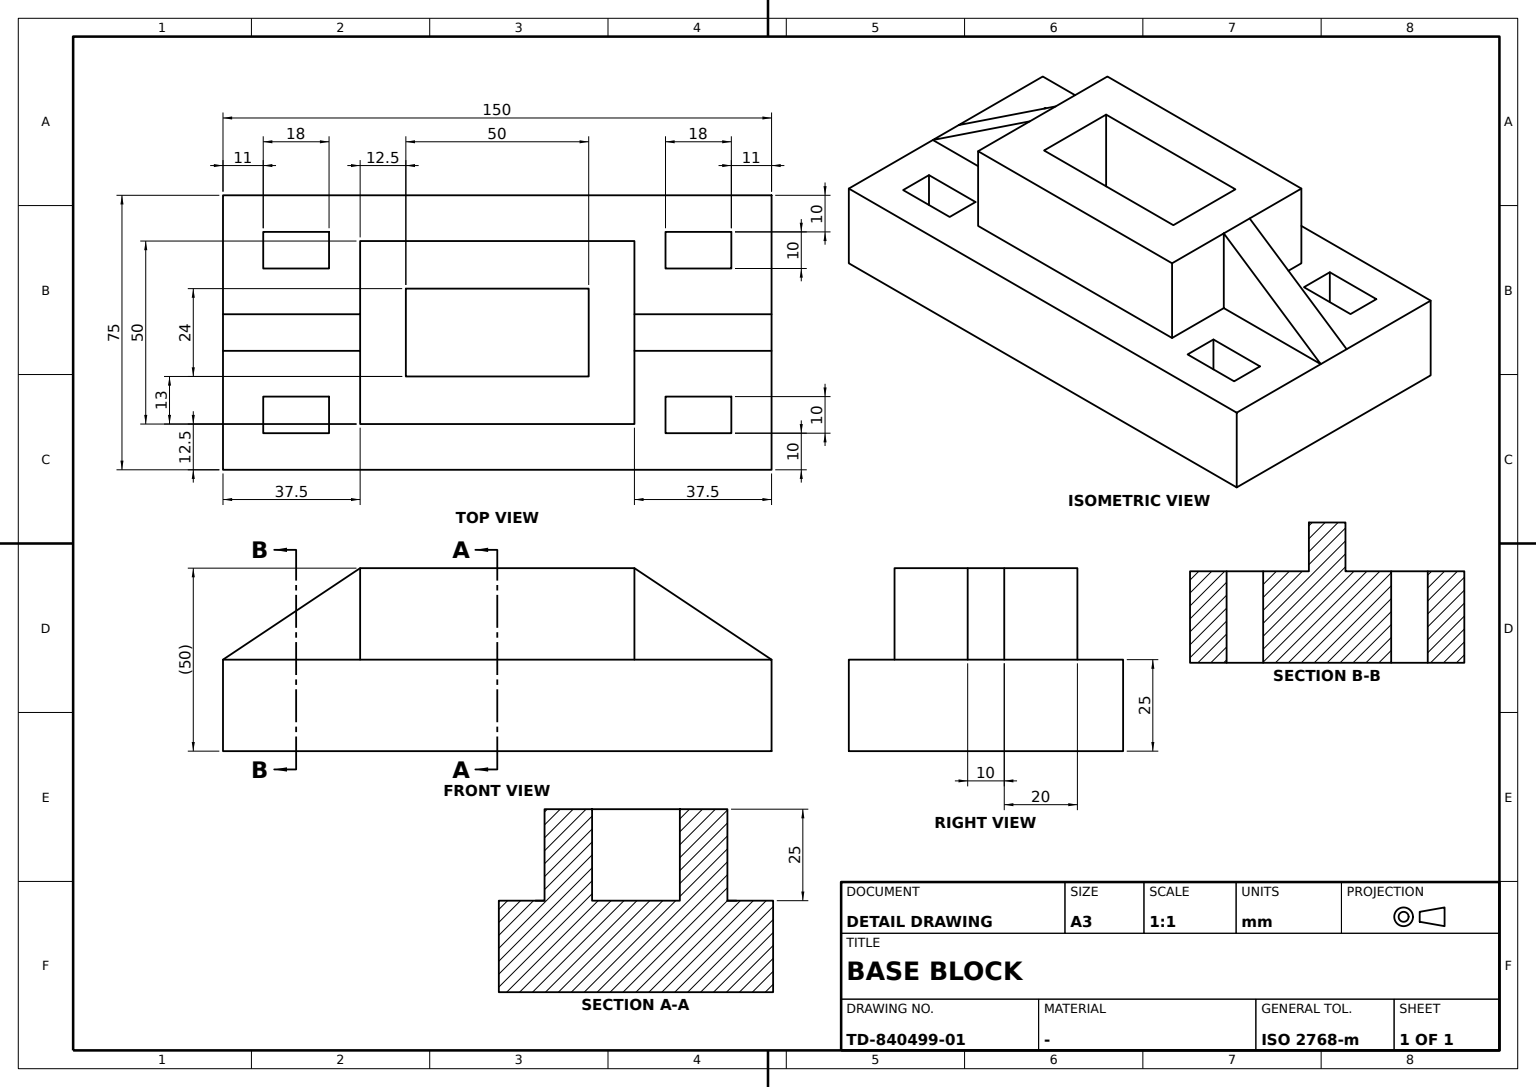
ISO-10303-21;
HEADER;
FILE_DESCRIPTION((''),'2;1');
FILE_NAME('','',(''),(''),'','','');
FILE_SCHEMA(('AUTOMOTIVE_DESIGN'));
ENDSEC;
DATA;
#1=APPLICATION_CONTEXT('');
#2=PRODUCT_CONTEXT('',#1,'mechanical');
#3=PRODUCT('','','',(#2));
#4=PRODUCT_DEFINITION_FORMATION('','',#3);
#5=PRODUCT_DEFINITION_CONTEXT('',#1,'design');
#6=PRODUCT_DEFINITION('','',#4,#5);
#7=PRODUCT_DEFINITION_SHAPE('','',#6);
#8=(LENGTH_UNIT()NAMED_UNIT(*)SI_UNIT(.MILLI.,.METRE.));
#9=(NAMED_UNIT(*)PLANE_ANGLE_UNIT()SI_UNIT($,.RADIAN.));
#10=(NAMED_UNIT(*)SI_UNIT($,.STERADIAN.)SOLID_ANGLE_UNIT());
#11=UNCERTAINTY_MEASURE_WITH_UNIT(LENGTH_MEASURE(0.005),#8,'distance_accuracy_value','');
#12=(GEOMETRIC_REPRESENTATION_CONTEXT(3)GLOBAL_UNCERTAINTY_ASSIGNED_CONTEXT((#11))GLOBAL_UNIT_ASSIGNED_CONTEXT((#8,#9,#10))REPRESENTATION_CONTEXT('',''));
#13=CARTESIAN_POINT('',(-46.,17.5,25.));
#14=VERTEX_POINT('',#13);
#15=CARTESIAN_POINT('',(-64.,17.5,25.));
#16=VERTEX_POINT('',#15);
#17=CARTESIAN_POINT('',(64.,17.5,25.));
#18=DIRECTION('',(-1.,0.,0.));
#19=VECTOR('',#18,1000.);
#20=LINE('',#17,#19);
#21=EDGE_CURVE('',#14,#16,#20,.T.);
#22=ORIENTED_EDGE('',*,*,#21,.F.);
#23=CARTESIAN_POINT('',(-46.,17.5,0.));
#24=VERTEX_POINT('',#23);
#25=DIRECTION('',(0.,0.,-1.));
#26=VECTOR('',#25,1000.);
#27=LINE('',#13,#26);
#28=EDGE_CURVE('',#14,#24,#27,.T.);
#29=ORIENTED_EDGE('',*,*,#28,.T.);
#30=CARTESIAN_POINT('',(-64.,17.5,0.));
#31=VERTEX_POINT('',#30);
#32=CARTESIAN_POINT('',(64.,17.5,0.));
#33=LINE('',#32,#19);
#34=EDGE_CURVE('',#24,#31,#33,.T.);
#35=ORIENTED_EDGE('',*,*,#34,.T.);
#36=LINE('',#15,#26);
#37=EDGE_CURVE('',#16,#31,#36,.T.);
#38=ORIENTED_EDGE('',*,*,#37,.F.);
#39=EDGE_LOOP('',(#22,#29,#35,#38));
#40=FACE_BOUND('',#39,.T.);
#41=DIRECTION('',(0.,-1.,0.));
#42=AXIS2_PLACEMENT_3D('',#17,#41,#18);
#43=PLANE('',#42);
#44=ADVANCED_FACE('',(#40),#43,.F.);
#45=VERTEX_POINT('',#17);
#46=CARTESIAN_POINT('',(46.,17.5,25.));
#47=VERTEX_POINT('',#46);
#48=EDGE_CURVE('',#45,#47,#20,.T.);
#49=ORIENTED_EDGE('',*,*,#48,.F.);
#50=VERTEX_POINT('',#32);
#51=LINE('',#17,#26);
#52=EDGE_CURVE('',#45,#50,#51,.T.);
#53=ORIENTED_EDGE('',*,*,#52,.T.);
#54=CARTESIAN_POINT('',(46.,17.5,0.));
#55=VERTEX_POINT('',#54);
#56=EDGE_CURVE('',#50,#55,#33,.T.);
#57=ORIENTED_EDGE('',*,*,#56,.T.);
#58=LINE('',#46,#26);
#59=EDGE_CURVE('',#47,#55,#58,.T.);
#60=ORIENTED_EDGE('',*,*,#59,.F.);
#61=EDGE_LOOP('',(#49,#53,#57,#60));
#62=FACE_BOUND('',#61,.T.);
#63=ADVANCED_FACE('',(#62),#43,.F.);
#64=CARTESIAN_POINT('',(75.,37.5,0.));
#65=VERTEX_POINT('',#64);
#66=CARTESIAN_POINT('',(75.,37.5,25.));
#67=VERTEX_POINT('',#66);
#68=DIRECTION('',(0.,0.,1.));
#69=VECTOR('',#68,1000.);
#70=LINE('',#64,#69);
#71=EDGE_CURVE('',#65,#67,#70,.T.);
#72=ORIENTED_EDGE('',*,*,#71,.F.);
#73=CARTESIAN_POINT('',(-75.,37.5,0.));
#74=VERTEX_POINT('',#73);
#75=CARTESIAN_POINT('',(0.,37.5,0.));
#76=DIRECTION('',(1.,0.,0.));
#77=VECTOR('',#76,1000.);
#78=LINE('',#75,#77);
#79=EDGE_CURVE('',#74,#65,#78,.T.);
#80=ORIENTED_EDGE('',*,*,#79,.F.);
#81=CARTESIAN_POINT('',(-75.,37.5,25.));
#82=VERTEX_POINT('',#81);
#83=LINE('',#73,#69);
#84=EDGE_CURVE('',#74,#82,#83,.T.);
#85=ORIENTED_EDGE('',*,*,#84,.T.);
#86=CARTESIAN_POINT('',(0.,37.5,25.));
#87=LINE('',#86,#77);
#88=EDGE_CURVE('',#82,#67,#87,.T.);
#89=ORIENTED_EDGE('',*,*,#88,.T.);
#90=EDGE_LOOP('',(#72,#80,#85,#89));
#91=FACE_BOUND('',#90,.T.);
#92=AXIS2_PLACEMENT_3D('',#73,#41,#76);
#93=PLANE('',#92);
#94=ADVANCED_FACE('',(#91),#93,.F.);
#95=CARTESIAN_POINT('',(75.,-5.,25.));
#96=VERTEX_POINT('',#95);
#97=CARTESIAN_POINT('',(75.,5.,25.));
#98=VERTEX_POINT('',#97);
#99=DIRECTION('',(0.,1.,0.));
#100=VECTOR('',#99,1000.);
#101=LINE('',#66,#100);
#102=EDGE_CURVE('',#96,#98,#101,.T.);
#103=ORIENTED_EDGE('',*,*,#102,.T.);
#104=CARTESIAN_POINT('',(37.5,5.,50.));
#105=VERTEX_POINT('',#104);
#106=CARTESIAN_POINT('',(34.615385,5.,51.923077));
#107=DIRECTION('',(0.832050294,0.,-0.554700196));
#108=VECTOR('',#107,1000.);
#109=LINE('',#106,#108);
#110=EDGE_CURVE('',#105,#98,#109,.T.);
#111=ORIENTED_EDGE('',*,*,#110,.F.);
#112=CARTESIAN_POINT('',(37.5,-5.,50.));
#113=VERTEX_POINT('',#112);
#114=CARTESIAN_POINT('',(37.5,0.,50.));
#115=LINE('',#114,#100);
#116=EDGE_CURVE('',#113,#105,#115,.T.);
#117=ORIENTED_EDGE('',*,*,#116,.F.);
#118=CARTESIAN_POINT('',(34.615385,-5.,51.923077));
#119=LINE('',#118,#108);
#120=EDGE_CURVE('',#113,#96,#119,.T.);
#121=ORIENTED_EDGE('',*,*,#120,.T.);
#122=EDGE_LOOP('',(#103,#111,#117,#121));
#123=FACE_BOUND('',#122,.T.);
#124=DIRECTION('',(0.554700196,0.,0.832050294));
#125=AXIS2_PLACEMENT_3D('',#114,#124,#107);
#126=PLANE('',#125);
#127=ADVANCED_FACE('',(#123),#126,.T.);
#128=ORIENTED_EDGE('',*,*,#79,.T.);
#129=CARTESIAN_POINT('',(75.,-37.5,0.));
#130=VERTEX_POINT('',#129);
#131=CARTESIAN_POINT('',(75.,0.,0.));
#132=VECTOR('',#41,1000.);
#133=LINE('',#131,#132);
#134=EDGE_CURVE('',#65,#130,#133,.T.);
#135=ORIENTED_EDGE('',*,*,#134,.T.);
#136=CARTESIAN_POINT('',(-75.,-37.5,0.));
#137=VERTEX_POINT('',#136);
#138=CARTESIAN_POINT('',(0.,-37.5,0.));
#139=LINE('',#138,#19);
#140=EDGE_CURVE('',#130,#137,#139,.T.);
#141=ORIENTED_EDGE('',*,*,#140,.T.);
#142=CARTESIAN_POINT('',(-75.,0.,0.));
#143=LINE('',#142,#100);
#144=EDGE_CURVE('',#137,#74,#143,.T.);
#145=ORIENTED_EDGE('',*,*,#144,.T.);
#146=EDGE_LOOP('',(#128,#135,#141,#145));
#147=FACE_BOUND('',#146,.T.);
#148=CARTESIAN_POINT('',(64.,-27.5,0.));
#149=VERTEX_POINT('',#148);
#150=CARTESIAN_POINT('',(46.,-27.5,0.));
#151=VERTEX_POINT('',#150);
#152=LINE('',#148,#19);
#153=EDGE_CURVE('',#149,#151,#152,.T.);
#154=ORIENTED_EDGE('',*,*,#153,.F.);
#155=CARTESIAN_POINT('',(64.,-17.5,0.));
#156=VERTEX_POINT('',#155);
#157=CARTESIAN_POINT('',(64.,27.5,0.));
#158=LINE('',#157,#132);
#159=EDGE_CURVE('',#156,#149,#158,.T.);
#160=ORIENTED_EDGE('',*,*,#159,.F.);
#161=CARTESIAN_POINT('',(46.,-17.5,0.));
#162=VERTEX_POINT('',#161);
#163=LINE('',#161,#77);
#164=EDGE_CURVE('',#162,#156,#163,.T.);
#165=ORIENTED_EDGE('',*,*,#164,.F.);
#166=LINE('',#54,#100);
#167=EDGE_CURVE('',#151,#162,#166,.T.);
#168=ORIENTED_EDGE('',*,*,#167,.F.);
#169=EDGE_LOOP('',(#154,#160,#165,#168));
#170=FACE_BOUND('',#169,.T.);
#171=VERTEX_POINT('',#157);
#172=EDGE_CURVE('',#171,#50,#158,.T.);
#173=ORIENTED_EDGE('',*,*,#172,.F.);
#174=CARTESIAN_POINT('',(46.,27.5,0.));
#175=VERTEX_POINT('',#174);
#176=LINE('',#174,#77);
#177=EDGE_CURVE('',#175,#171,#176,.T.);
#178=ORIENTED_EDGE('',*,*,#177,.F.);
#179=EDGE_CURVE('',#55,#175,#166,.T.);
#180=ORIENTED_EDGE('',*,*,#179,.F.);
#181=ORIENTED_EDGE('',*,*,#56,.F.);
#182=EDGE_LOOP('',(#173,#178,#180,#181));
#183=FACE_BOUND('',#182,.T.);
#184=CARTESIAN_POINT('',(-46.,-17.5,0.));
#185=VERTEX_POINT('',#184);
#186=CARTESIAN_POINT('',(-46.,-27.5,0.));
#187=VERTEX_POINT('',#186);
#188=CARTESIAN_POINT('',(-46.,27.5,0.));
#189=LINE('',#188,#132);
#190=EDGE_CURVE('',#185,#187,#189,.T.);
#191=ORIENTED_EDGE('',*,*,#190,.F.);
#192=CARTESIAN_POINT('',(-64.,-17.5,0.));
#193=VERTEX_POINT('',#192);
#194=EDGE_CURVE('',#193,#185,#163,.T.);
#195=ORIENTED_EDGE('',*,*,#194,.F.);
#196=CARTESIAN_POINT('',(-64.,-27.5,0.));
#197=VERTEX_POINT('',#196);
#198=LINE('',#30,#100);
#199=EDGE_CURVE('',#197,#193,#198,.T.);
#200=ORIENTED_EDGE('',*,*,#199,.F.);
#201=EDGE_CURVE('',#187,#197,#152,.T.);
#202=ORIENTED_EDGE('',*,*,#201,.F.);
#203=EDGE_LOOP('',(#191,#195,#200,#202));
#204=FACE_BOUND('',#203,.T.);
#205=VERTEX_POINT('',#188);
#206=EDGE_CURVE('',#205,#24,#189,.T.);
#207=ORIENTED_EDGE('',*,*,#206,.F.);
#208=CARTESIAN_POINT('',(-64.,27.5,0.));
#209=VERTEX_POINT('',#208);
#210=EDGE_CURVE('',#209,#205,#176,.T.);
#211=ORIENTED_EDGE('',*,*,#210,.F.);
#212=EDGE_CURVE('',#31,#209,#198,.T.);
#213=ORIENTED_EDGE('',*,*,#212,.F.);
#214=ORIENTED_EDGE('',*,*,#34,.F.);
#215=EDGE_LOOP('',(#207,#211,#213,#214));
#216=FACE_BOUND('',#215,.T.);
#217=CARTESIAN_POINT('',(0.,0.,0.));
#218=AXIS2_PLACEMENT_3D('',#217,#68,#76);
#219=PLANE('',#218);
#220=ADVANCED_FACE('',(#147,#170,#183,#204,#216),#219,.F.);
#221=CARTESIAN_POINT('',(25.,-12.,50.));
#222=VERTEX_POINT('',#221);
#223=CARTESIAN_POINT('',(-25.,-12.,50.));
#224=VERTEX_POINT('',#223);
#225=CARTESIAN_POINT('',(0.,-12.,50.));
#226=LINE('',#225,#19);
#227=EDGE_CURVE('',#222,#224,#226,.T.);
#228=ORIENTED_EDGE('',*,*,#227,.T.);
#229=CARTESIAN_POINT('',(-25.,12.,50.));
#230=VERTEX_POINT('',#229);
#231=CARTESIAN_POINT('',(-25.,0.,50.));
#232=LINE('',#231,#100);
#233=EDGE_CURVE('',#224,#230,#232,.T.);
#234=ORIENTED_EDGE('',*,*,#233,.T.);
#235=CARTESIAN_POINT('',(25.,12.,50.));
#236=VERTEX_POINT('',#235);
#237=CARTESIAN_POINT('',(0.,12.,50.));
#238=LINE('',#237,#77);
#239=EDGE_CURVE('',#230,#236,#238,.T.);
#240=ORIENTED_EDGE('',*,*,#239,.T.);
#241=CARTESIAN_POINT('',(25.,0.,50.));
#242=LINE('',#241,#132);
#243=EDGE_CURVE('',#236,#222,#242,.T.);
#244=ORIENTED_EDGE('',*,*,#243,.T.);
#245=EDGE_LOOP('',(#228,#234,#240,#244));
#246=FACE_BOUND('',#245,.T.);
#247=CARTESIAN_POINT('',(-37.5,-5.,50.));
#248=VERTEX_POINT('',#247);
#249=CARTESIAN_POINT('',(-37.5,5.,50.));
#250=VERTEX_POINT('',#249);
#251=CARTESIAN_POINT('',(-37.5,0.,50.));
#252=LINE('',#251,#100);
#253=EDGE_CURVE('',#248,#250,#252,.T.);
#254=ORIENTED_EDGE('',*,*,#253,.F.);
#255=CARTESIAN_POINT('',(-37.5,-25.,50.));
#256=VERTEX_POINT('',#255);
#257=EDGE_CURVE('',#256,#248,#252,.T.);
#258=ORIENTED_EDGE('',*,*,#257,.F.);
#259=CARTESIAN_POINT('',(37.5,-25.,50.));
#260=VERTEX_POINT('',#259);
#261=CARTESIAN_POINT('',(0.,-25.,50.));
#262=LINE('',#261,#19);
#263=EDGE_CURVE('',#260,#256,#262,.T.);
#264=ORIENTED_EDGE('',*,*,#263,.F.);
#265=LINE('',#114,#132);
#266=EDGE_CURVE('',#113,#260,#265,.T.);
#267=ORIENTED_EDGE('',*,*,#266,.F.);
#268=ORIENTED_EDGE('',*,*,#116,.T.);
#269=CARTESIAN_POINT('',(37.5,25.,50.));
#270=VERTEX_POINT('',#269);
#271=EDGE_CURVE('',#270,#105,#265,.T.);
#272=ORIENTED_EDGE('',*,*,#271,.F.);
#273=CARTESIAN_POINT('',(-37.5,25.,50.));
#274=VERTEX_POINT('',#273);
#275=CARTESIAN_POINT('',(0.,25.,50.));
#276=LINE('',#275,#77);
#277=EDGE_CURVE('',#274,#270,#276,.T.);
#278=ORIENTED_EDGE('',*,*,#277,.F.);
#279=EDGE_CURVE('',#250,#274,#252,.T.);
#280=ORIENTED_EDGE('',*,*,#279,.F.);
#281=EDGE_LOOP('',(#254,#258,#264,#267,#268,#272,#278,#280));
#282=FACE_BOUND('',#281,.T.);
#283=CARTESIAN_POINT('',(0.,0.,50.));
#284=AXIS2_PLACEMENT_3D('',#283,#68,#76);
#285=PLANE('',#284);
#286=ADVANCED_FACE('',(#246,#282),#285,.T.);
#287=CARTESIAN_POINT('',(46.,27.5,25.));
#288=VERTEX_POINT('',#287);
#289=CARTESIAN_POINT('',(64.,27.5,25.));
#290=VERTEX_POINT('',#289);
#291=LINE('',#287,#77);
#292=EDGE_CURVE('',#288,#290,#291,.T.);
#293=ORIENTED_EDGE('',*,*,#292,.F.);
#294=LINE('',#287,#26);
#295=EDGE_CURVE('',#288,#175,#294,.T.);
#296=ORIENTED_EDGE('',*,*,#295,.T.);
#297=ORIENTED_EDGE('',*,*,#177,.T.);
#298=LINE('',#289,#26);
#299=EDGE_CURVE('',#290,#171,#298,.T.);
#300=ORIENTED_EDGE('',*,*,#299,.F.);
#301=EDGE_LOOP('',(#293,#296,#297,#300));
#302=FACE_BOUND('',#301,.T.);
#303=AXIS2_PLACEMENT_3D('',#287,#99,#76);
#304=PLANE('',#303);
#305=ADVANCED_FACE('',(#302),#304,.F.);
#306=CARTESIAN_POINT('',(-25.,12.,25.));
#307=VERTEX_POINT('',#306);
#308=CARTESIAN_POINT('',(25.,12.,25.));
#309=VERTEX_POINT('',#308);
#310=CARTESIAN_POINT('',(0.,12.,25.));
#311=LINE('',#310,#77);
#312=EDGE_CURVE('',#307,#309,#311,.T.);
#313=ORIENTED_EDGE('',*,*,#312,.T.);
#314=LINE('',#308,#69);
#315=EDGE_CURVE('',#309,#236,#314,.T.);
#316=ORIENTED_EDGE('',*,*,#315,.T.);
#317=ORIENTED_EDGE('',*,*,#239,.F.);
#318=LINE('',#306,#69);
#319=EDGE_CURVE('',#307,#230,#318,.T.);
#320=ORIENTED_EDGE('',*,*,#319,.F.);
#321=EDGE_LOOP('',(#313,#316,#317,#320));
#322=FACE_BOUND('',#321,.T.);
#323=AXIS2_PLACEMENT_3D('',#306,#41,#76);
#324=PLANE('',#323);
#325=ADVANCED_FACE('',(#322),#324,.T.);
#326=CARTESIAN_POINT('',(-64.,27.5,25.));
#327=VERTEX_POINT('',#326);
#328=LINE('',#15,#100);
#329=EDGE_CURVE('',#16,#327,#328,.T.);
#330=ORIENTED_EDGE('',*,*,#329,.F.);
#331=ORIENTED_EDGE('',*,*,#37,.T.);
#332=ORIENTED_EDGE('',*,*,#212,.T.);
#333=LINE('',#326,#26);
#334=EDGE_CURVE('',#327,#209,#333,.T.);
#335=ORIENTED_EDGE('',*,*,#334,.F.);
#336=EDGE_LOOP('',(#330,#331,#332,#335));
#337=FACE_BOUND('',#336,.T.);
#338=AXIS2_PLACEMENT_3D('',#15,#18,#99);
#339=PLANE('',#338);
#340=ADVANCED_FACE('',(#337),#339,.F.);
#341=CARTESIAN_POINT('',(-25.,-12.,25.));
#342=VERTEX_POINT('',#341);
#343=LINE('',#341,#69);
#344=EDGE_CURVE('',#342,#224,#343,.T.);
#345=ORIENTED_EDGE('',*,*,#344,.F.);
#346=CARTESIAN_POINT('',(-25.,0.,25.));
#347=LINE('',#346,#100);
#348=EDGE_CURVE('',#342,#307,#347,.T.);
#349=ORIENTED_EDGE('',*,*,#348,.T.);
#350=ORIENTED_EDGE('',*,*,#319,.T.);
#351=ORIENTED_EDGE('',*,*,#233,.F.);
#352=EDGE_LOOP('',(#345,#349,#350,#351));
#353=FACE_BOUND('',#352,.T.);
#354=AXIS2_PLACEMENT_3D('',#341,#76,#99);
#355=PLANE('',#354);
#356=ADVANCED_FACE('',(#353),#355,.T.);
#357=CARTESIAN_POINT('',(-37.5,-5.,25.));
#358=VERTEX_POINT('',#357);
#359=CARTESIAN_POINT('',(-75.,-5.,25.));
#360=VERTEX_POINT('',#359);
#361=CARTESIAN_POINT('',(0.,-5.,25.));
#362=LINE('',#361,#19);
#363=EDGE_CURVE('',#358,#360,#362,.T.);
#364=ORIENTED_EDGE('',*,*,#363,.F.);
#365=CARTESIAN_POINT('',(-37.5,-5.,0.));
#366=LINE('',#365,#26);
#367=EDGE_CURVE('',#248,#358,#366,.T.);
#368=ORIENTED_EDGE('',*,*,#367,.F.);
#369=CARTESIAN_POINT('',(-34.615385,-5.,51.923077));
#370=DIRECTION('',(0.832050294,0.,0.554700196));
#371=VECTOR('',#370,1000.);
#372=LINE('',#369,#371);
#373=EDGE_CURVE('',#360,#248,#372,.T.);
#374=ORIENTED_EDGE('',*,*,#373,.F.);
#375=EDGE_LOOP('',(#364,#368,#374));
#376=FACE_BOUND('',#375,.T.);
#377=CARTESIAN_POINT('',(0.,-5.,0.));
#378=AXIS2_PLACEMENT_3D('',#377,#99,#18);
#379=PLANE('',#378);
#380=ADVANCED_FACE('',(#376),#379,.F.);
#381=CARTESIAN_POINT('',(37.5,-25.,25.));
#382=VERTEX_POINT('',#381);
#383=LINE('',#381,#69);
#384=EDGE_CURVE('',#382,#260,#383,.T.);
#385=ORIENTED_EDGE('',*,*,#384,.F.);
#386=CARTESIAN_POINT('',(37.5,-5.,25.));
#387=VERTEX_POINT('',#386);
#388=CARTESIAN_POINT('',(37.5,0.,25.));
#389=LINE('',#388,#132);
#390=EDGE_CURVE('',#387,#382,#389,.T.);
#391=ORIENTED_EDGE('',*,*,#390,.F.);
#392=CARTESIAN_POINT('',(37.5,-5.,0.));
#393=LINE('',#392,#69);
#394=EDGE_CURVE('',#387,#113,#393,.T.);
#395=ORIENTED_EDGE('',*,*,#394,.T.);
#396=ORIENTED_EDGE('',*,*,#266,.T.);
#397=EDGE_LOOP('',(#385,#391,#395,#396));
#398=FACE_BOUND('',#397,.T.);
#399=CARTESIAN_POINT('',(37.5,25.,25.));
#400=AXIS2_PLACEMENT_3D('',#399,#18,#41);
#401=PLANE('',#400);
#402=ADVANCED_FACE('',(#398),#401,.F.);
#403=CARTESIAN_POINT('',(-37.5,5.,25.));
#404=VERTEX_POINT('',#403);
#405=CARTESIAN_POINT('',(-37.5,5.,0.));
#406=LINE('',#405,#26);
#407=EDGE_CURVE('',#250,#404,#406,.T.);
#408=ORIENTED_EDGE('',*,*,#407,.F.);
#409=ORIENTED_EDGE('',*,*,#279,.T.);
#410=CARTESIAN_POINT('',(-37.5,25.,25.));
#411=VERTEX_POINT('',#410);
#412=LINE('',#410,#69);
#413=EDGE_CURVE('',#411,#274,#412,.T.);
#414=ORIENTED_EDGE('',*,*,#413,.F.);
#415=CARTESIAN_POINT('',(-37.5,0.,25.));
#416=LINE('',#415,#100);
#417=EDGE_CURVE('',#404,#411,#416,.T.);
#418=ORIENTED_EDGE('',*,*,#417,.F.);
#419=EDGE_LOOP('',(#408,#409,#414,#418));
#420=FACE_BOUND('',#419,.T.);
#421=CARTESIAN_POINT('',(-37.5,-25.,25.));
#422=AXIS2_PLACEMENT_3D('',#421,#76,#99);
#423=PLANE('',#422);
#424=ADVANCED_FACE('',(#420),#423,.F.);
#425=CARTESIAN_POINT('',(46.,-27.5,25.));
#426=VERTEX_POINT('',#425);
#427=LINE('',#425,#26);
#428=EDGE_CURVE('',#426,#151,#427,.T.);
#429=ORIENTED_EDGE('',*,*,#428,.F.);
#430=CARTESIAN_POINT('',(64.,-27.5,25.));
#431=VERTEX_POINT('',#430);
#432=LINE('',#430,#19);
#433=EDGE_CURVE('',#431,#426,#432,.T.);
#434=ORIENTED_EDGE('',*,*,#433,.F.);
#435=LINE('',#430,#26);
#436=EDGE_CURVE('',#431,#149,#435,.T.);
#437=ORIENTED_EDGE('',*,*,#436,.T.);
#438=ORIENTED_EDGE('',*,*,#153,.T.);
#439=EDGE_LOOP('',(#429,#434,#437,#438));
#440=FACE_BOUND('',#439,.T.);
#441=AXIS2_PLACEMENT_3D('',#430,#41,#18);
#442=PLANE('',#441);
#443=ADVANCED_FACE('',(#440),#442,.F.);
#444=CARTESIAN_POINT('',(-46.,-27.5,25.));
#445=VERTEX_POINT('',#444);
#446=CARTESIAN_POINT('',(-64.,-27.5,25.));
#447=VERTEX_POINT('',#446);
#448=EDGE_CURVE('',#445,#447,#432,.T.);
#449=ORIENTED_EDGE('',*,*,#448,.F.);
#450=LINE('',#444,#26);
#451=EDGE_CURVE('',#445,#187,#450,.T.);
#452=ORIENTED_EDGE('',*,*,#451,.T.);
#453=ORIENTED_EDGE('',*,*,#201,.T.);
#454=LINE('',#446,#26);
#455=EDGE_CURVE('',#447,#197,#454,.T.);
#456=ORIENTED_EDGE('',*,*,#455,.F.);
#457=EDGE_LOOP('',(#449,#452,#453,#456));
#458=FACE_BOUND('',#457,.T.);
#459=ADVANCED_FACE('',(#458),#442,.F.);
#460=ORIENTED_EDGE('',*,*,#194,.T.);
#461=CARTESIAN_POINT('',(-46.,-17.5,25.));
#462=VERTEX_POINT('',#461);
#463=LINE('',#461,#26);
#464=EDGE_CURVE('',#462,#185,#463,.T.);
#465=ORIENTED_EDGE('',*,*,#464,.F.);
#466=CARTESIAN_POINT('',(-64.,-17.5,25.));
#467=VERTEX_POINT('',#466);
#468=CARTESIAN_POINT('',(46.,-17.5,25.));
#469=LINE('',#468,#77);
#470=EDGE_CURVE('',#467,#462,#469,.T.);
#471=ORIENTED_EDGE('',*,*,#470,.F.);
#472=LINE('',#466,#26);
#473=EDGE_CURVE('',#467,#193,#472,.T.);
#474=ORIENTED_EDGE('',*,*,#473,.T.);
#475=EDGE_LOOP('',(#460,#465,#471,#474));
#476=FACE_BOUND('',#475,.T.);
#477=AXIS2_PLACEMENT_3D('',#468,#99,#76);
#478=PLANE('',#477);
#479=ADVANCED_FACE('',(#476),#478,.F.);
#480=ORIENTED_EDGE('',*,*,#312,.F.);
#481=ORIENTED_EDGE('',*,*,#348,.F.);
#482=CARTESIAN_POINT('',(25.,-12.,25.));
#483=VERTEX_POINT('',#482);
#484=CARTESIAN_POINT('',(0.,-12.,25.));
#485=LINE('',#484,#19);
#486=EDGE_CURVE('',#483,#342,#485,.T.);
#487=ORIENTED_EDGE('',*,*,#486,.F.);
#488=CARTESIAN_POINT('',(25.,0.,25.));
#489=LINE('',#488,#132);
#490=EDGE_CURVE('',#309,#483,#489,.T.);
#491=ORIENTED_EDGE('',*,*,#490,.F.);
#492=EDGE_LOOP('',(#480,#481,#487,#491));
#493=FACE_BOUND('',#492,.T.);
#494=CARTESIAN_POINT('',(0.,0.,25.));
#495=AXIS2_PLACEMENT_3D('',#494,#68,#76);
#496=PLANE('',#495);
#497=ADVANCED_FACE('',(#493),#496,.T.);
#498=LINE('',#289,#132);
#499=EDGE_CURVE('',#290,#45,#498,.T.);
#500=ORIENTED_EDGE('',*,*,#499,.F.);
#501=ORIENTED_EDGE('',*,*,#299,.T.);
#502=ORIENTED_EDGE('',*,*,#172,.T.);
#503=ORIENTED_EDGE('',*,*,#52,.F.);
#504=EDGE_LOOP('',(#500,#501,#502,#503));
#505=FACE_BOUND('',#504,.T.);
#506=AXIS2_PLACEMENT_3D('',#289,#76,#41);
#507=PLANE('',#506);
#508=ADVANCED_FACE('',(#505),#507,.F.);
#509=VERTEX_POINT('',#399);
#510=CARTESIAN_POINT('',(0.,25.,25.));
#511=LINE('',#510,#77);
#512=EDGE_CURVE('',#411,#509,#511,.T.);
#513=ORIENTED_EDGE('',*,*,#512,.F.);
#514=ORIENTED_EDGE('',*,*,#413,.T.);
#515=ORIENTED_EDGE('',*,*,#277,.T.);
#516=LINE('',#399,#69);
#517=EDGE_CURVE('',#509,#270,#516,.T.);
#518=ORIENTED_EDGE('',*,*,#517,.F.);
#519=EDGE_LOOP('',(#513,#514,#515,#518));
#520=FACE_BOUND('',#519,.T.);
#521=AXIS2_PLACEMENT_3D('',#410,#41,#76);
#522=PLANE('',#521);
#523=ADVANCED_FACE('',(#520),#522,.F.);
#524=ORIENTED_EDGE('',*,*,#367,.T.);
#525=VERTEX_POINT('',#421);
#526=EDGE_CURVE('',#525,#358,#416,.T.);
#527=ORIENTED_EDGE('',*,*,#526,.F.);
#528=LINE('',#421,#69);
#529=EDGE_CURVE('',#525,#256,#528,.T.);
#530=ORIENTED_EDGE('',*,*,#529,.T.);
#531=ORIENTED_EDGE('',*,*,#257,.T.);
#532=EDGE_LOOP('',(#524,#527,#530,#531));
#533=FACE_BOUND('',#532,.T.);
#534=ADVANCED_FACE('',(#533),#423,.F.);
#535=ORIENTED_EDGE('',*,*,#295,.F.);
#536=LINE('',#46,#100);
#537=EDGE_CURVE('',#47,#288,#536,.T.);
#538=ORIENTED_EDGE('',*,*,#537,.F.);
#539=ORIENTED_EDGE('',*,*,#59,.T.);
#540=ORIENTED_EDGE('',*,*,#179,.T.);
#541=EDGE_LOOP('',(#535,#538,#539,#540));
#542=FACE_BOUND('',#541,.T.);
#543=AXIS2_PLACEMENT_3D('',#46,#18,#99);
#544=PLANE('',#543);
#545=ADVANCED_FACE('',(#542),#544,.F.);
#546=ORIENTED_EDGE('',*,*,#486,.T.);
#547=ORIENTED_EDGE('',*,*,#344,.T.);
#548=ORIENTED_EDGE('',*,*,#227,.F.);
#549=LINE('',#482,#69);
#550=EDGE_CURVE('',#483,#222,#549,.T.);
#551=ORIENTED_EDGE('',*,*,#550,.F.);
#552=EDGE_LOOP('',(#546,#547,#548,#551));
#553=FACE_BOUND('',#552,.T.);
#554=AXIS2_PLACEMENT_3D('',#482,#99,#18);
#555=PLANE('',#554);
#556=ADVANCED_FACE('',(#553),#555,.T.);
#557=ORIENTED_EDGE('',*,*,#428,.T.);
#558=ORIENTED_EDGE('',*,*,#167,.T.);
#559=VERTEX_POINT('',#468);
#560=LINE('',#468,#26);
#561=EDGE_CURVE('',#559,#162,#560,.T.);
#562=ORIENTED_EDGE('',*,*,#561,.F.);
#563=EDGE_CURVE('',#426,#559,#536,.T.);
#564=ORIENTED_EDGE('',*,*,#563,.F.);
#565=EDGE_LOOP('',(#557,#558,#562,#564));
#566=FACE_BOUND('',#565,.T.);
#567=ADVANCED_FACE('',(#566),#544,.F.);
#568=CARTESIAN_POINT('',(-46.,27.5,25.));
#569=VERTEX_POINT('',#568);
#570=LINE('',#568,#26);
#571=EDGE_CURVE('',#569,#205,#570,.T.);
#572=ORIENTED_EDGE('',*,*,#571,.T.);
#573=ORIENTED_EDGE('',*,*,#206,.T.);
#574=ORIENTED_EDGE('',*,*,#28,.F.);
#575=LINE('',#568,#132);
#576=EDGE_CURVE('',#569,#14,#575,.T.);
#577=ORIENTED_EDGE('',*,*,#576,.F.);
#578=EDGE_LOOP('',(#572,#573,#574,#577));
#579=FACE_BOUND('',#578,.T.);
#580=AXIS2_PLACEMENT_3D('',#568,#76,#41);
#581=PLANE('',#580);
#582=ADVANCED_FACE('',(#579),#581,.F.);
#583=ORIENTED_EDGE('',*,*,#464,.T.);
#584=ORIENTED_EDGE('',*,*,#190,.T.);
#585=ORIENTED_EDGE('',*,*,#451,.F.);
#586=EDGE_CURVE('',#462,#445,#575,.T.);
#587=ORIENTED_EDGE('',*,*,#586,.F.);
#588=EDGE_LOOP('',(#583,#584,#585,#587));
#589=FACE_BOUND('',#588,.T.);
#590=ADVANCED_FACE('',(#589),#581,.F.);
#591=ORIENTED_EDGE('',*,*,#550,.T.);
#592=ORIENTED_EDGE('',*,*,#243,.F.);
#593=ORIENTED_EDGE('',*,*,#315,.F.);
#594=ORIENTED_EDGE('',*,*,#490,.T.);
#595=EDGE_LOOP('',(#591,#592,#593,#594));
#596=FACE_BOUND('',#595,.T.);
#597=AXIS2_PLACEMENT_3D('',#308,#18,#41);
#598=PLANE('',#597);
#599=ADVANCED_FACE('',(#596),#598,.T.);
#600=ORIENTED_EDGE('',*,*,#159,.T.);
#601=ORIENTED_EDGE('',*,*,#436,.F.);
#602=CARTESIAN_POINT('',(64.,-17.5,25.));
#603=VERTEX_POINT('',#602);
#604=EDGE_CURVE('',#603,#431,#498,.T.);
#605=ORIENTED_EDGE('',*,*,#604,.F.);
#606=LINE('',#602,#26);
#607=EDGE_CURVE('',#603,#156,#606,.T.);
#608=ORIENTED_EDGE('',*,*,#607,.T.);
#609=EDGE_LOOP('',(#600,#601,#605,#608));
#610=FACE_BOUND('',#609,.T.);
#611=ADVANCED_FACE('',(#610),#507,.F.);
#612=CARTESIAN_POINT('',(-75.,-37.5,25.));
#613=VERTEX_POINT('',#612);
#614=LINE('',#136,#69);
#615=EDGE_CURVE('',#137,#613,#614,.T.);
#616=ORIENTED_EDGE('',*,*,#615,.T.);
#617=CARTESIAN_POINT('',(-75.,0.,25.));
#618=LINE('',#617,#100);
#619=EDGE_CURVE('',#613,#360,#618,.T.);
#620=ORIENTED_EDGE('',*,*,#619,.T.);
#621=CARTESIAN_POINT('',(-75.,5.,25.));
#622=VERTEX_POINT('',#621);
#623=EDGE_CURVE('',#360,#622,#618,.T.);
#624=ORIENTED_EDGE('',*,*,#623,.T.);
#625=EDGE_CURVE('',#622,#82,#618,.T.);
#626=ORIENTED_EDGE('',*,*,#625,.T.);
#627=ORIENTED_EDGE('',*,*,#84,.F.);
#628=ORIENTED_EDGE('',*,*,#144,.F.);
#629=EDGE_LOOP('',(#616,#620,#624,#626,#627,#628));
#630=FACE_BOUND('',#629,.T.);
#631=AXIS2_PLACEMENT_3D('',#136,#76,#99);
#632=PLANE('',#631);
#633=ADVANCED_FACE('',(#630),#632,.F.);
#634=ORIENTED_EDGE('',*,*,#110,.T.);
#635=CARTESIAN_POINT('',(37.5,5.,25.));
#636=VERTEX_POINT('',#635);
#637=CARTESIAN_POINT('',(0.,5.,25.));
#638=LINE('',#637,#19);
#639=EDGE_CURVE('',#98,#636,#638,.T.);
#640=ORIENTED_EDGE('',*,*,#639,.T.);
#641=CARTESIAN_POINT('',(37.5,5.,0.));
#642=LINE('',#641,#69);
#643=EDGE_CURVE('',#636,#105,#642,.T.);
#644=ORIENTED_EDGE('',*,*,#643,.T.);
#645=EDGE_LOOP('',(#634,#640,#644));
#646=FACE_BOUND('',#645,.T.);
#647=CARTESIAN_POINT('',(0.,5.,0.));
#648=AXIS2_PLACEMENT_3D('',#647,#99,#18);
#649=PLANE('',#648);
#650=ADVANCED_FACE('',(#646),#649,.T.);
#651=EDGE_CURVE('',#559,#603,#469,.T.);
#652=ORIENTED_EDGE('',*,*,#651,.F.);
#653=ORIENTED_EDGE('',*,*,#561,.T.);
#654=ORIENTED_EDGE('',*,*,#164,.T.);
#655=ORIENTED_EDGE('',*,*,#607,.F.);
#656=EDGE_LOOP('',(#652,#653,#654,#655));
#657=FACE_BOUND('',#656,.T.);
#658=ADVANCED_FACE('',(#657),#478,.F.);
#659=ORIENTED_EDGE('',*,*,#571,.F.);
#660=EDGE_CURVE('',#327,#569,#291,.T.);
#661=ORIENTED_EDGE('',*,*,#660,.F.);
#662=ORIENTED_EDGE('',*,*,#334,.T.);
#663=ORIENTED_EDGE('',*,*,#210,.T.);
#664=EDGE_LOOP('',(#659,#661,#662,#663));
#665=FACE_BOUND('',#664,.T.);
#666=ADVANCED_FACE('',(#665),#304,.F.);
#667=ORIENTED_EDGE('',*,*,#199,.T.);
#668=ORIENTED_EDGE('',*,*,#473,.F.);
#669=EDGE_CURVE('',#447,#467,#328,.T.);
#670=ORIENTED_EDGE('',*,*,#669,.F.);
#671=ORIENTED_EDGE('',*,*,#455,.T.);
#672=EDGE_LOOP('',(#667,#668,#670,#671));
#673=FACE_BOUND('',#672,.T.);
#674=ADVANCED_FACE('',(#673),#339,.F.);
#675=CARTESIAN_POINT('',(-34.615385,5.,51.923077));
#676=LINE('',#675,#371);
#677=EDGE_CURVE('',#622,#250,#676,.T.);
#678=ORIENTED_EDGE('',*,*,#677,.T.);
#679=ORIENTED_EDGE('',*,*,#407,.T.);
#680=EDGE_CURVE('',#404,#622,#638,.T.);
#681=ORIENTED_EDGE('',*,*,#680,.T.);
#682=EDGE_LOOP('',(#678,#679,#681));
#683=FACE_BOUND('',#682,.T.);
#684=ADVANCED_FACE('',(#683),#649,.T.);
#685=ORIENTED_EDGE('',*,*,#448,.T.);
#686=ORIENTED_EDGE('',*,*,#669,.T.);
#687=ORIENTED_EDGE('',*,*,#470,.T.);
#688=ORIENTED_EDGE('',*,*,#586,.T.);
#689=EDGE_LOOP('',(#685,#686,#687,#688));
#690=FACE_BOUND('',#689,.T.);
#691=CARTESIAN_POINT('',(75.,-37.5,25.));
#692=VERTEX_POINT('',#691);
#693=CARTESIAN_POINT('',(75.,0.,25.));
#694=LINE('',#693,#132);
#695=EDGE_CURVE('',#96,#692,#694,.T.);
#696=ORIENTED_EDGE('',*,*,#695,.F.);
#697=EDGE_CURVE('',#96,#387,#362,.T.);
#698=ORIENTED_EDGE('',*,*,#697,.T.);
#699=ORIENTED_EDGE('',*,*,#390,.T.);
#700=CARTESIAN_POINT('',(0.,-25.,25.));
#701=LINE('',#700,#19);
#702=EDGE_CURVE('',#382,#525,#701,.T.);
#703=ORIENTED_EDGE('',*,*,#702,.T.);
#704=ORIENTED_EDGE('',*,*,#526,.T.);
#705=ORIENTED_EDGE('',*,*,#363,.T.);
#706=ORIENTED_EDGE('',*,*,#619,.F.);
#707=CARTESIAN_POINT('',(0.,-37.5,25.));
#708=LINE('',#707,#19);
#709=EDGE_CURVE('',#692,#613,#708,.T.);
#710=ORIENTED_EDGE('',*,*,#709,.F.);
#711=EDGE_LOOP('',(#696,#698,#699,#703,#704,#705,#706,#710));
#712=FACE_BOUND('',#711,.T.);
#713=ORIENTED_EDGE('',*,*,#563,.T.);
#714=ORIENTED_EDGE('',*,*,#651,.T.);
#715=ORIENTED_EDGE('',*,*,#604,.T.);
#716=ORIENTED_EDGE('',*,*,#433,.T.);
#717=EDGE_LOOP('',(#713,#714,#715,#716));
#718=FACE_BOUND('',#717,.T.);
#719=ADVANCED_FACE('',(#690,#712,#718),#496,.T.);
#720=ORIENTED_EDGE('',*,*,#102,.F.);
#721=ORIENTED_EDGE('',*,*,#695,.T.);
#722=LINE('',#129,#69);
#723=EDGE_CURVE('',#130,#692,#722,.T.);
#724=ORIENTED_EDGE('',*,*,#723,.F.);
#725=ORIENTED_EDGE('',*,*,#134,.F.);
#726=ORIENTED_EDGE('',*,*,#71,.T.);
#727=EDGE_CURVE('',#67,#98,#694,.T.);
#728=ORIENTED_EDGE('',*,*,#727,.T.);
#729=EDGE_LOOP('',(#720,#721,#724,#725,#726,#728));
#730=FACE_BOUND('',#729,.T.);
#731=AXIS2_PLACEMENT_3D('',#64,#18,#41);
#732=PLANE('',#731);
#733=ADVANCED_FACE('',(#730),#732,.F.);
#734=ORIENTED_EDGE('',*,*,#709,.T.);
#735=ORIENTED_EDGE('',*,*,#615,.F.);
#736=ORIENTED_EDGE('',*,*,#140,.F.);
#737=ORIENTED_EDGE('',*,*,#723,.T.);
#738=EDGE_LOOP('',(#734,#735,#736,#737));
#739=FACE_BOUND('',#738,.T.);
#740=AXIS2_PLACEMENT_3D('',#129,#99,#18);
#741=PLANE('',#740);
#742=ADVANCED_FACE('',(#739),#741,.F.);
#743=ORIENTED_EDGE('',*,*,#697,.F.);
#744=ORIENTED_EDGE('',*,*,#120,.F.);
#745=ORIENTED_EDGE('',*,*,#394,.F.);
#746=EDGE_LOOP('',(#743,#744,#745));
#747=FACE_BOUND('',#746,.T.);
#748=ADVANCED_FACE('',(#747),#379,.F.);
#749=ORIENTED_EDGE('',*,*,#529,.F.);
#750=ORIENTED_EDGE('',*,*,#702,.F.);
#751=ORIENTED_EDGE('',*,*,#384,.T.);
#752=ORIENTED_EDGE('',*,*,#263,.T.);
#753=EDGE_LOOP('',(#749,#750,#751,#752));
#754=FACE_BOUND('',#753,.T.);
#755=AXIS2_PLACEMENT_3D('',#381,#99,#18);
#756=PLANE('',#755);
#757=ADVANCED_FACE('',(#754),#756,.F.);
#758=EDGE_CURVE('',#509,#636,#389,.T.);
#759=ORIENTED_EDGE('',*,*,#758,.F.);
#760=ORIENTED_EDGE('',*,*,#517,.T.);
#761=ORIENTED_EDGE('',*,*,#271,.T.);
#762=ORIENTED_EDGE('',*,*,#643,.F.);
#763=EDGE_LOOP('',(#759,#760,#761,#762));
#764=FACE_BOUND('',#763,.T.);
#765=ADVANCED_FACE('',(#764),#401,.F.);
#766=ORIENTED_EDGE('',*,*,#677,.F.);
#767=ORIENTED_EDGE('',*,*,#623,.F.);
#768=ORIENTED_EDGE('',*,*,#373,.T.);
#769=ORIENTED_EDGE('',*,*,#253,.T.);
#770=EDGE_LOOP('',(#766,#767,#768,#769));
#771=FACE_BOUND('',#770,.T.);
#772=DIRECTION('',(-0.554700196,0.,0.832050294));
#773=AXIS2_PLACEMENT_3D('',#617,#772,#370);
#774=PLANE('',#773);
#775=ADVANCED_FACE('',(#771),#774,.T.);
#776=ORIENTED_EDGE('',*,*,#512,.T.);
#777=ORIENTED_EDGE('',*,*,#758,.T.);
#778=ORIENTED_EDGE('',*,*,#639,.F.);
#779=ORIENTED_EDGE('',*,*,#727,.F.);
#780=ORIENTED_EDGE('',*,*,#88,.F.);
#781=ORIENTED_EDGE('',*,*,#625,.F.);
#782=ORIENTED_EDGE('',*,*,#680,.F.);
#783=ORIENTED_EDGE('',*,*,#417,.T.);
#784=EDGE_LOOP('',(#776,#777,#778,#779,#780,#781,#782,#783));
#785=FACE_BOUND('',#784,.T.);
#786=ORIENTED_EDGE('',*,*,#48,.T.);
#787=ORIENTED_EDGE('',*,*,#537,.T.);
#788=ORIENTED_EDGE('',*,*,#292,.T.);
#789=ORIENTED_EDGE('',*,*,#499,.T.);
#790=EDGE_LOOP('',(#786,#787,#788,#789));
#791=FACE_BOUND('',#790,.T.);
#792=ORIENTED_EDGE('',*,*,#660,.T.);
#793=ORIENTED_EDGE('',*,*,#576,.T.);
#794=ORIENTED_EDGE('',*,*,#21,.T.);
#795=ORIENTED_EDGE('',*,*,#329,.T.);
#796=EDGE_LOOP('',(#792,#793,#794,#795));
#797=FACE_BOUND('',#796,.T.);
#798=ADVANCED_FACE('',(#785,#791,#797),#496,.T.);
#799=CLOSED_SHELL('',(#44,#63,#94,#127,#220,#286,#305,#325,#340,#356,#380,#402,#424,#443,#459,#479,#497,#508,#523,#534,#545,#556,#567,#582,#590,#599,#611,#633,#650,#658,#666,#674,#684,#719,#733,#742,#748,#757,#765,#775,#798));
#800=MANIFOLD_SOLID_BREP('',#799);
#801=ADVANCED_BREP_SHAPE_REPRESENTATION('',(#800),#12);
#802=SHAPE_DEFINITION_REPRESENTATION(#7,#801);
ENDSEC;
END-ISO-10303-21;
